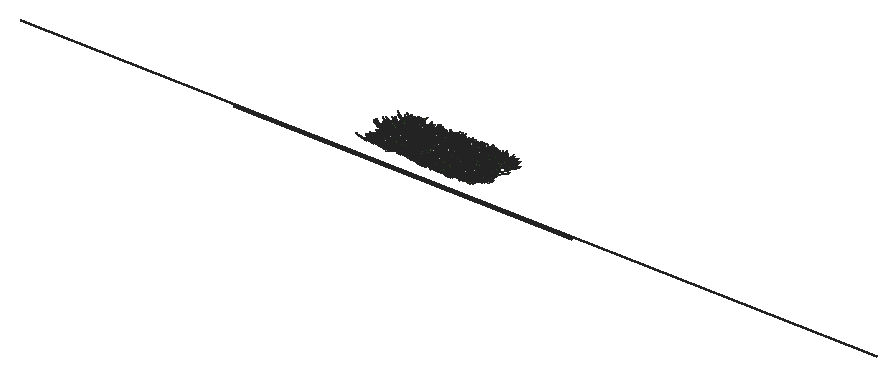
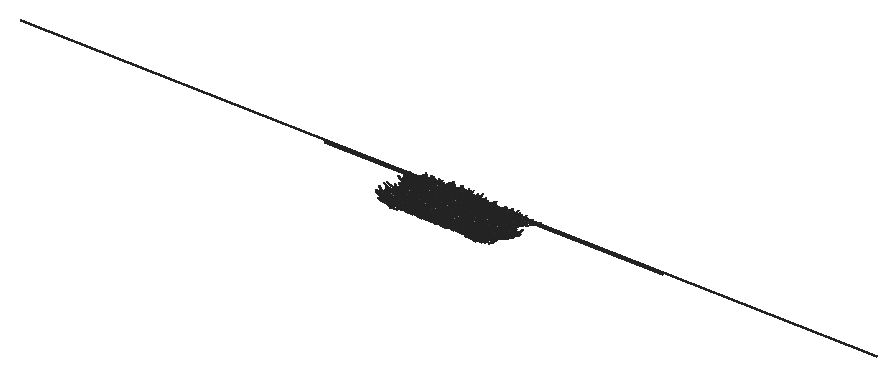
# SketchUp Ruby script. Lengths in inches.
U = 1.inch
M = Sketchup.active_model
def pt(a) = Geom::Point3d.new(a.map { |v| v * U })
def face(e, loops, mat)
  f = e.add_face(loops[0].map { |a| pt(a) })
  loops[1..].each { |l| e.add_face(l.map { |a| pt(a) }).erase! }
  f.material = f.back_material = mat if mat
  f
end
# faces: each face lists its corners as indices into pts; further lists are holes
def faces(e, pts, list, mat = nil) = list.each { |f| face(e, (f[0].is_a?(Array) ? f : [f]).map { |l| l.map { |i| pts[i] } }, mat) }
# xy, xz, yz: faces in a plane at the given z, y or x. An outline is a flat list of corners, or four numbers for a rectangle; further outlines are holes
def ring(l) = l.size == 4 ? [[l[0], l[1]], [l[2], l[1]], [l[2], l[3]], [l[0], l[3]]] : l.each_slice(2).to_a
def flat(e, list, mat, &to3) = list.each { |f| face(e, (f[0].is_a?(Array) ? f : [f]).map { |l| ring(l).map { |u, v| to3.(u, v) } }, mat) }
def xy(e, z, list, mat = nil) = flat(e, list, mat) { |x, y| [x, y, z] }
def xz(e, y, list, mat = nil) = flat(e, list, mat) { |x, z| [x, y, z] }
def yz(e, x, list, mat = nil) = flat(e, list, mat) { |y, z| [x, y, z] }
def lines(e, pts, list) = list.each { |a, b| e.add_line(pt(pts[a]), pt(pts[b])) }
# prism: a flat outline (further loops are holes) pulled along v
def prism(e, loops, v, mat = nil)
  f = face(e, loops, mat); d = Geom::Vector3d.new(v.map { |x| x * U })
  f.pushpull(f.normal.samedirection?(d) ? d.length : -d.length)
end
def box(e, o, s, mat = nil) = prism(e, [[o, [o[0] + s[0], o[1], o[2]], [o[0] + s[0], o[1] + s[1], o[2]], [o[0], o[1] + s[1], o[2]]]], [0, 0, s[2]], mat)
def at(x, y, z, deg = 0) = Geom::Transformation.translation(pt([x, y, z])) * Geom::Transformation.rotation(ORIGIN, Z_AXIS, deg.degrees)
def axes(o, x, y, z) = Geom::Transformation.new([*x, 0, *y, 0, *z, 0, *pt(o).to_a, 1])
def part(name) = M.definitions.add(name)
# library, detail: a bought-in or finely detailed component or shape, given as its bounding box
def library(name, o, s) = part(name).tap { |d| box(d.entities, o, s) }
def detail(e, o, s) = box(e.add_group.entities, o, s)
def put(e, d, t, mat = nil) = e.add_instance(d, t).tap { |i| i.material = mat if mat }
def group(e, t, mat = nil) = e.add_group.tap { |g| g.transformation = t; g.material = mat if mat }.entities
root = M.entities
M.materials.add("Material82").color = [68, 110, 58]
M.materials.add("Material83").color = [48, 90, 38]
M.materials.add("Material84").color = [68, 110, 48]
M.materials.add("Material85").color = [48, 90, 48]
M.materials.add("Material86").color = [58, 110, 58]
M.materials.add("Material87").color = [58, 90, 38]
M.materials.add("Material88").color = [68, 100, 58]
M.materials.add("Material89").color = [48, 100, 38]
c1 = part("grass00")
p = [[-0.6875,0.15,0],[-0.56,0.08,5.52],[-0.04,0.03,2.76],[0.48,-0.02,0],[0.35,-0.02,5.52],[-0.1,-0.14,5.52],
  [-0.12,0.65,8.37],[-0.42,0.65,8.37]]
faces(c1.entities,p,[[0,1,2,3],[3,2,4],[1,5,2],[5,4,2],[1,6,5],[4,5,6],[7,6,1]])
c2 = part("Group16\#1")
put(c2.entities,c1,axes([1.44,-0.61,-0.01],[0.05352,0.12609,0],[-0.10704,0.04543,0.07239],[0.06664,-0.02828,0.11628]),"Material85")
put(c2.entities,c1,axes([0.76,-0.15,-0.01],[0.04676,0.24062,0],[-0.23162,0.04501,0.06642],[0.0652,-0.01267,0.23595]),"Material82")
put(c2.entities,c1,axes([0.79,0.01,-0.01],[-0.00606,0.34651,0],[-0.34381,-0.00602,0.0432],[0.04319,0.00076,0.34386]))
put(c2.entities,c1,axes([1,0.23,-0.01],[-0.07192,0.31144,0],[-0.28722,-0.06632,0.1236],[0.12043,0.02781,0.29478]),"Material84")
put(c2.entities,c1,axes([1.66,0.77,-0.01],[-0.13828,0.29651,0],[-0.21551,-0.1005,0.22471],[0.20365,0.09498,0.23779]),"Material89")
put(c2.entities,c1,axes([0.6875,0.52,-0.01],[-0.18126,0.24051,0],[-0.22746,-0.17142,0.09788],[0.07817,0.05891,0.28481]),"Material84")
put(c2.entities,c1,axes([0.68,0.78,-0.01],[-0.215,0.18688,0],[-0.12385,-0.14248,0.21334],[0.13995,0.16101,0.18878]),"Material82")
put(c2.entities,c1,axes([0.56,1,-0.01],[-0.13756,0.07624,0],[-0.06159,-0.11112,0.0927],[0.04494,0.08108,0.12705]),"Material84")
put(c2.entities,c1,axes([0.2,0.64,-0.01],[-0.23729,0.07254,0],[-0.05711,-0.18681,0.153],[0.04473,0.14632,0.19535]),"Material89")
put(c2.entities,c1,axes([0.0625,0.72,-0.01],[-0.28874,0.02525,0],[-0.02179,-0.24916,0.14647],[0.01276,0.14591,0.25012]),"Material82")
put(c2.entities,c1,axes([-0.08,0.62,-0.01],[-0.34089,-0.04187,0],[0.03255,-0.26504,0.216],[-0.02633,0.21439,0.26703]),"Material89")
put(c2.entities,c1,axes([-0.34,0.98,-0.01],[-0.14314,-0.0493,0],[0.04397,-0.12769,0.06843],[-0.02228,0.0647,0.13505]),"Material89")
put(c2.entities,c1,axes([-0.87,1.45,-0.01],[-0.23488,-0.14114,0],[0.13761,-0.22901,0.06087],[-0.03135,0.05217,0.26717]))
put(c2.entities,c1,axes([-0.72,0.77,-0.01],[-0.14208,-0.13251,0],[0.07209,-0.0773,0.16301],[-0.11118,0.11922,0.1057]),"Material89")
put(c2.entities,c1,axes([-0.62,0.43,-0.01],[-0.14845,-0.21203,0],[0.18654,-0.13061,0.12304],[-0.10079,0.07057,0.22772]),"Material82")
put(c2.entities,c1,axes([-0.68,0.29,-0.01],[-0.13639,-0.32136,0],[0.31723,-0.13464,0.05579],[-0.05136,0.0218,0.34462]),"Material83")
put(c2.entities,c1,axes([-0.64,0.125,-0.01],[-0.0458,-0.23569,0],[0.22124,-0.043,0.08276],[-0.08124,0.01579,0.22538]),"Material86")
put(c2.entities,c1,axes([-1.6,-0.03,-0.01],[0.00576,-0.32897,0],[0.27526,0.00482,0.18018],[-0.18015,-0.00315,0.2753]),"Material84")
put(c2.entities,c1,axes([-1.36,-0.31,-0.01],[0.05718,-0.24765,0],[0.18172,0.04196,0.17267],[-0.16825,-0.03885,0.1865]),"Material89")
put(c2.entities,c1,axes([-1.54,-0.72,-0.01],[0.06537,-0.14017,0],[0.13555,0.06321,0.03939],[-0.0357,-0.01665,0.14956]))
put(c2.entities,c1,axes([-1.19,-0.9,-0.01],[0.09597,-0.12735,0],[0.11214,0.08451,0.07557],[-0.06035,-0.04548,0.14042]),"Material88")
put(c2.entities,c1,axes([-0.47,-0.54,-0.01],[0.11588,-0.10072,0],[0.0618,0.0711,0.12124],[-0.07953,-0.0915,0.0942]))
put(c2.entities,c1,axes([-0.47,-0.84,-0.01],[0.11927,-0.0661,0],[0.06603,0.11913,0.00646],[-0.00313,-0.00565,0.13621]),"Material84")
put(c2.entities,c1,axes([-0.38,-1.24,-0.01],[0.28037,-0.08571,0],[0.0618,0.20215,0.20315],[-0.05939,-0.19428,0.21139]),"Material88")
put(c2.entities,c1,axes([-0.06,-0.66,-0.01],[0.22719,-0.01987,0],[0.01247,0.14255,0.17758],[-0.01547,-0.17691,0.1431]),"Material87")
put(c2.entities,c1,axes([0.11,-0.89,-0.01],[0.14882,0.01828,0],[-0.01058,0.08611,0.12229],[0.01491,-0.12138,0.08676]),"Material85")
put(c2.entities,c1,axes([0.25,-0.72,-0.01],[0.20481,0.07053,0],[-0.06206,0.18022,0.10291],[0.03351,-0.0973,0.1906]),"Material85")
put(c2.entities,c1,axes([0.85,-1.42,-0.01],[0.16481,0.09904,0],[-0.09472,0.15762,0.05616],[0.02893,-0.04814,0.18389]),"Material84")
put(c2.entities,c1,axes([1.01,-1.09,-0.01],[0.21858,0.20385,0],[-0.17495,0.1876,0.15339],[0.10462,-0.11218,0.25652]),"Material89")
put(c2.entities,c1,axes([1.01,-0.71,-0.01],[0.08733,0.12473,0],[-0.06445,0.04512,0.13037],[0.1068,-0.07477,0.07867]),"Material85")
c3 = part("Group15\#1")
put(c3.entities,c2,at(0,0,0))
c4 = part("3darcstudiotree_grass00\#1")
put(c4.entities,c3,at(0,0,0))
xz(root,273.41,[[1674.99,-39.125,1897.28,-38.61],[1534.73,-37.86,2096.97,-37.24]])
put(root,c4,axes([1803.56,281.3125,-34.17],[3.22982,-1.36398,0],[2.52221,0.92889,-0.01281],[0.05669,0.02088,1.56626]))
put(root,c4,axes([1811.6875,281.07,-34.17],[0.45304,1.69594,0],[-3.37186,0.14009,-0.01763],[-0.11097,0.00461,1.60818]))
put(root,c4,axes([1801.04,281.26,-34.17],[-2.98133,1.10226,0],[-2.6348,-1.10837,-0.04557],[-0.21161,-0.08902,1.96028]))
put(root,c4,axes([1793.37,281.49,-34.17],[0.75696,1.65896,0],[-4.64105,0.32936,-0.03105],[-0.12997,0.00922,1.50318]))
put(root,c4,axes([1821.67,281.36,-34.17],[-1.86859,1.14232,0],[-3.14905,-0.80116,-0.00439],[-0.02189,-0.00557,1.66469]))
put(root,c4,axes([1767.47,282.96,-34.17],[3.31562,-0.63662,0],[1.81859,1.47309,-0.02466],[0.05194,0.04207,1.49812]))
put(root,c4,axes([1817.85,282.6,-34.17],[2.60331,1.05125,0],[-2.58261,0.9947,-0.01838],[-0.08057,0.03103,1.65818]))
put(root,c4,axes([1783.02,282.9375,-34.17],[4.09444,0.12503,0],[-0.31641,1.61154,-0.0417],[-0.02006,0.10219,1.91485]))
put(root,c4,axes([1804.3,283.15,-34.17],[3.14565,-0.76847,0],[1.85222,1.17921,-0.00486],[0.01386,0.00882,1.42853]))
put(root,c4,axes([1786.66,282.67,-34.17],[-0.14266,1.36173,0],[-4.10184,-0.06683,-0.00296],[-0.01424,-0.00023,1.47961]))
put(root,c4,axes([1770.84,282.6,-34.17],[-3.65106,0.9561,0],[-2.55118,-1.5152,-0.05111],[-0.12576,-0.07469,1.53759]))
put(root,c4,axes([1798.7,282.95,-34.17],[-3.45178,0.2701,0],[-0.90786,-1.80446,-0.05548],[-0.0508,-0.10098,1.6451]))
put(root,c4,axes([1775.57,283.58,-34.17],[3.35024,-0.43777,0],[1.10858,1.31952,-0.03222],[0.06859,0.08164,1.78787]))
put(root,c4,axes([1762.07,283.2,-34.17],[-4.08016,-0.15242,0],[0.34321,-1.42893,-0.02721],[0.0124,-0.05162,1.31849]))
put(root,c4,axes([1820.89,283.29,-34.17],[-0.10583,1.54224,0],[-3.7996,-0.04055,-0.00627],[-0.03571,-0.00038,1.62459]))
put(root,c4,axes([1792.28,283.65,-34.17],[-2.56709,-0.87628,0],[2.75862,-1.25691,-0.00422],[0.01164,-0.0053,1.33295]))
put(root,c4,axes([1810.66,283.9,-34.17],[2.94971,1.39882,0],[-3.26889,1.07209,-0.02991],[-0.14108,0.04627,1.95467]))
put(root,c4,axes([1787.83,284.71,-34.17],[3.68364,0.44666,0],[-1.28613,1.64968,-0.02064],[-0.02718,0.03487,1.46981]))
put(root,c4,axes([1804.67,285.1,-34.17],[1.53079,-1.5017,0],[4.19952,0.6658,-0.01772],[0.08663,0.01374,1.7874]))
put(root,c4,axes([1765.65,284.68,-34.17],[-0.8053,1.43922,0],[-4.1788,-0.36366,-0.05256],[-0.20936,-0.01822,1.30827]))
put(root,c4,axes([1800.85,285.36,-34.17],[1.13972,-1.41461,0],[4.50389,0.56436,-0.03698],[0.18209,0.02282,1.82987]))
put(root,c4,axes([1782.94,285.26,-34.17],[3.61655,0.77067,0],[-2.16585,1.58076,-0.05913],[-0.11484,0.08382,1.39517]))
put(root,c4,axes([1794.16,285.29,-34.17],[-1.56362,-1.21345,0],[3.6466,-0.73082,-0.00876],[0.03709,-0.00743,1.45672]))
put(root,c4,axes([1823.15,285.4,-34.17],[-3.61232,0.8121,0],[-2.24589,-1.55373,-0.01918],[-0.05035,-0.03483,1.80194]))
put(root,c4,axes([1814.34,286.01,-34.17],[3.57437,0.42668,0],[-1.04232,1.35805,-0.0422],[-0.08519,0.111,1.87907]))
put(root,c4,axes([1776.02,286.11,-34.17],[2.52987,0.96809,0],[-2.35442,0.95693,-0.00683],[-0.03278,0.01332,1.74693]))
put(root,c4,axes([1773,285.88,-34.17],[0.40934,1.39565,0],[-3.638,0.16595,-0.04522],[-0.26335,0.01201,1.60941]))
put(root,c4,axes([1812.32,285.87,-34.17],[-3.36311,0.85521,0],[-1.93534,-1.1837,-0.01497],[-0.0443,-0.0271,1.4615]))
put(root,c4,axes([1817.17,286.72,-34.17],[-0.65586,-1.46962,0],[4.60144,-0.31938,-0.05842],[0.32577,-0.02261,1.98292]))
put(root,c4,axes([1826.3,286.73,-34.17],[-3.01218,-1.1682,0],[2.32929,-0.93411,-0.00764],[0.03903,-0.01565,1.81511]))
put(root,c4,axes([1776.07,286.96,-34.17],[0.10079,1.33733,0],[-4.05045,0.04748,-0.05613],[-0.28184,0.0033,1.5259]))
put(root,c4,axes([1821.84,287.11,-34.17],[-0.80891,1.58211,0],[-4.50454,-0.3582,-0.03197],[-0.1625,-0.01292,1.78572]))
put(root,c4,axes([1811.23,287.18,-34.17],[-2.18902,1.07825,0],[-2.9207,-0.92221,-0.02462],[-0.13408,-0.04234,1.95656]))
put(root,c4,axes([1769.99,287.61,-34.17],[-2.79747,-0.82267,0],[2.4,-1.26929,-0.00029],[0.00098,-0.00052,1.69542]))
put(root,c4,axes([1795.17,287.51,-34.17],[0.20899,1.64265,0],[-4.27343,0.08456,-0.03261],[-0.1888,0.00374,1.85888]))
put(root,c4,axes([1784,287.79,-34.17],[-3.83423,-0.51133,0],[1.38691,-1.61748,-0.06149],[0.1095,-0.1277,1.80385]))
put(root,c4,axes([1806.43,288.25,-34.17],[0.38628,-1.42854,0],[3.50239,0.14729,-0.04937],[0.32013,0.01346,1.72169]))
put(root,c4,axes([1766.97,287.69,-34.17],[-1.21632,1.56365,0],[-3.36368,-0.40694,-0.03727],[-0.21338,-0.02582,1.57911]))
put(root,c4,axes([1789.53,287.77,-34.17],[-2.10873,0.99525,0],[-2.92476,-0.96381,-0.03387],[-0.14037,-0.04626,1.54303]))
put(root,c4,axes([1781.45,289.03,-34.17],[4.32757,-0.42653,0],[1.12297,1.77206,-0.03338],[0.0321,0.05066,1.37691]))
put(root,c4,axes([1801.32,288.3,-34.17],[-3.3677,0.38425,0],[-1.22656,-1.67195,-0.00573],[-0.0077,-0.0105,1.59925]))
put(root,c4,axes([1798.86,289.42,-34.17],[4.24203,-0.02956,0],[0.08072,1.80172,-0.02875],[0.00231,0.05162,1.55972]))
put(root,c4,axes([1779.08,289.23,-34.17],[-2.64283,-1.13535,0],[3.48014,-1.25993,-0.02326],[0.08818,-0.03192,1.82249]))
put(root,c4,axes([1816.71,289.62,-34.17],[1.16933,-1.48396,0],[3.883,0.47588,-0.02169],[0.1048,0.01284,1.54236]))
put(root,c4,axes([1804.05,289.61,-34.17],[3.86384,0.07818,0],[-0.23972,1.84255,-0.05168],[-0.01275,0.09801,1.68853]))
put(root,c4,axes([1789.375,289.94,-34.17],[3.33633,-0.58263,0],[1.85643,1.65335,-0.04981],[0.10311,0.09183,1.75709]))
put(root,c4,axes([1766.5,290.5,-34.17],[2.313,-1.43442,0],[2.99954,0.75225,-0.04064],[0.1888,0.04735,1.46692]))
put(root,c4,axes([1821.45,290.52,-34.17],[0.21445,-1.64927,0],[3.6182,0.07317,-0.01161],[0.06174,0.00125,1.44612]))
put(root,c4,axes([1792.65,290.38,-34.17],[2.09092,1.38555,0],[-3.43654,0.80658,-0.00188],[-0.01015,0.00238,1.87843]))
put(root,c4,axes([1811.67,290.52,-34.17],[-2.42754,-1.16571,0],[2.71881,-0.88058,-0.021],[0.08634,-0.02796,1.40308]))
put(root,c4,axes([1773.4,290.24,-34.17],[-2.97215,1.15542,0],[-3.15373,-1.26173,-0.01243],[-0.04576,-0.01831,1.76595]))
put(root,c4,axes([1812.72,291.39,-34.17],[3.8213,1.10557,0],[-2.37941,1.27911,-0.00415],[-0.01079,0.0058,1.32509]))
put(root,c4,axes([1766.01,291.5,-34.17],[3.43029,0.99275,0],[-1.97308,1.06035,-0.01519],[-0.04853,0.02608,1.34969]))
put(root,c4,axes([1820.98,291.5,-34.17],[-3.1974,-0.52057,0],[1.31873,-1.25975,-0.01181],[0.03016,-0.02882,1.73426]))
put(root,c4,axes([1800.07,291.51,-34.17],[-3.96689,-0.26306,0],[0.64548,-1.51387,-0.0114],[0.01279,-0.03,1.97478]))
put(root,c4,axes([1792.88,292.32,-34.17],[3.4734,-0.75241,0],[2.06047,1.47936,-0.02691],[0.07219,0.05183,1.78778]))
put(root,c4,axes([1778.53,292.4375,-34.17],[1.26532,-1.44178,0],[3.12553,0.42661,-0.00044],[0.00223,0.0003,1.32507]))
put(root,c4,axes([1769.97,292.03,-34.17],[2.61816,1.29298,0],[-2.60516,0.82044,-0.01421],[-0.06264,0.01973,1.40932]))
put(root,c4,axes([1787.01,292.6,-34.17],[2.17735,-1.14497,0],[3.55677,1.05197,-0.03529],[0.11494,0.03399,1.35654]))
put(root,c4,axes([1784.36,291.86,-34.17],[-3.45507,0.18922,0],[-0.60525,-1.7188,-0.02154],[-0.01288,-0.03658,1.4342]))
put(root,c4,axes([1806.86,291.99,-34.17],[0.41177,1.61489,0],[-3.5087,0.13914,-0.04963],[-0.27633,0.01096,1.47912]))
put(root,c4,axes([1816.5,292.23,-34.17],[-3.24054,-0.28468,0],[0.77392,-1.37016,-0.02543],[0.03342,-0.05916,1.61262]))
put(root,c4,axes([1778.15,293.65,-34.17],[3.40614,0.32781,0],[-0.81542,1.31776,-0.01459],[-0.02356,0.03807,1.75568]))
put(root,c4,axes([1823.04,293.92,-34.17],[4.64374,0.18316,0],[-0.43015,1.69615,-0.02551],[-0.01161,0.04577,1.48132]))
put(root,c4,axes([1789.8125,293.4,-34.17],[-3.50392,-0.27669,0],[0.88512,-1.7433,-0.02406],[0.02146,-0.04227,1.53532]))
put(root,c4,axes([1783.75,293.52,-34.17],[1.33968,1.52005,0],[-3.16755,0.43419,-0.01128],[-0.07711,0.01057,1.81963]))
put(root,c4,axes([1814.71,294.16,-34.17],[1.53865,-1.45346,0],[4.25105,0.69992,-0.03949],[0.18935,0.03118,1.7941]))
put(root,c4,axes([1769.93,294,-34.17],[-3.43052,-0.93956,0],[2.00829,-1.14045,-0.00375],[0.01479,-0.0084,1.82358]))
put(root,c4,axes([1798.24,294.53,-34.17],[-0.8562,-1.46222,0],[3.2715,-0.29793,-0.0292],[0.1741,-0.01586,1.53984]))
put(root,c4,axes([1805.19,294.38,-34.17],[-3.12873,-1.31633,0],[2.88309,-1.0658,-0.03051],[0.12402,-0.04585,1.65027]))
put(root,c4,axes([1764.82,294.17,-34.17],[1.08587,1.67228,0],[-4.264,0.43062,-0.00469],[-0.02209,0.00223,1.60422]))
put(root,c4,axes([1762.11,294.57,-34.17],[-2.42435,1.35441,0],[-3.23148,-0.89962,-0.04566],[-0.20763,-0.0578,1.65042]))
put(root,c4,axes([1795.18,294.8,-34.17],[-2.97303,0.61552,0],[-2.04085,-1.53313,-0.02543],[-0.06857,-0.05151,1.9093]))
put(root,c4,axes([1777.9375,295.45,-34.17],[0.04452,-1.40138,0],[3.5701,0.01764,-0.00992],[0.04898,0.00024,1.32167]))
put(root,c4,axes([1811.77,294.86,-34.17],[-4.30499,0.20084,0],[-0.50439,-1.68151,-0.02284],[-0.01208,-0.04026,1.44864]))
put(root,c4,axes([1801.41,295.68,-34.17],[-2.49551,-1.26471,0],[2.8619,-0.87828,-0.01663],[0.09126,-0.02801,1.89037]))
put(root,c4,axes([1782.125,296,-34.17],[3.17214,0.39156,0],[-1.05658,1.33127,-0.01935],[-0.04192,0.05282,1.92273]))
put(root,c4,axes([1760.46,296.01,-34.17],[3.52761,0.55067,0],[-1.26989,1.26523,-0.04887],[-0.1287,0.12823,1.85053]))
put(root,c4,axes([1768.47,296.8,-34.17],[3.22727,-0.96219,0],[2.40393,1.25403,-0.04167],[0.15655,0.08166,1.86151]))
put(root,c4,axes([1814.26,296.79,-34.17],[1.36885,-1.43158,0],[3.98655,0.59286,-0.04892],[0.27754,0.04127,1.93615]))
put(root,c4,axes([1809.48,296.19,-34.17],[-3.9685,0.8355,0],[-2.02289,-1.49439,-0.03463],[-0.09424,-0.06962,1.86049]))
put(root,c4,axes([1773.5,296.36,-34.17],[1.39622,1.62786,0],[-3.6301,0.48424,-0.04556],[-0.23124,0.03085,1.53888]))
put(root,c4,axes([1787.88,296.34,-34.17],[-4.01589,0.275,0],[-0.74615,-1.69466,-0.05401],[-0.03733,-0.08478,1.3206]))
put(root,c4,axes([1822.04,296.38,-34.17],[-3.10318,1.24143,0],[-2.60712,-1.01358,-0.05097],[-0.2393,-0.09303,1.80901]))
put(root,c4,axes([1803.88,296.39,-34.17],[0.17144,1.84869,0],[-4.60552,0.06643,-0.0182],[-0.07619,0.0011,1.44668]))
put(root,c4,axes([1794.84,296.81,-34.17],[2.02269,1.40625,0],[-2.88305,0.64496,-0.03898],[-0.27125,0.06068,1.98748]))
put(root,c4,axes([1765.61,297.63,-34.17],[0.48715,-1.38403,0],[3.63737,0.19912,-0.0013],[0.00869,0.00048,1.85519]))
put(root,c4,axes([1822.52,297.67,-34.17],[4.4529,0.04613,0],[-0.09862,1.48061,-0.04419],[-0.00818,0.12282,1.98467]))
put(root,c4,axes([1811.61,297.87,-34.17],[-1.73285,-1.40976,0],[3.20349,-0.61242,-0.03263],[0.20579,-0.03934,1.87]))
put(root,c4,axes([1789.68,297.76,-34.17],[0.25957,1.50579,0],[-3.94932,0.10588,-0.02807],[-0.1244,0.00334,1.3177]))
put(root,c4,axes([1778.29,298.47,-34.17],[3.60093,0.62069,0],[-1.54425,1.39338,-0.01451],[-0.03218,0.02903,1.59989]))
put(root,c4,axes([1817.85,298.41,-34.17],[-3.57377,-0.68668,0],[1.88387,-1.52489,-0.02869],[0.074,-0.0599,1.89824]))
put(root,c4,axes([1770.88,298.84,-34.17],[4.25337,0.6683,0],[-1.56461,1.54873,-0.01606],[-0.02903,0.02874,1.54782]))
put(root,c4,axes([1792.18,298.39,-34.17],[-2.10864,1.34219,0],[-3.56504,-0.87109,-0.01218],[-0.05259,-0.01285,1.59607]))
put(root,c4,axes([1781.2,298.36,-34.17],[-2.73949,1.39402,0],[-3.69271,-1.12865,-0.03455],[-0.12332,-0.03769,1.58129]))
put(root,c4,axes([1762.34,298.57,-34.17],[-4.29343,-0.7683,0],[1.85419,-1.61153,-0.00153],[0.00342,-0.00297,1.82565]))
put(root,c4,axes([1798.85,299.13,-34.17],[-0.26486,1.49696,0],[-3.89065,-0.10706,-0.02357],[-0.1242,-0.00342,1.54387]))
put(root,c4,axes([1766.81,299.89,-34.17],[2.27709,-1.12887,0],[2.96357,0.92974,-0.01848],[0.07518,0.02359,1.47553]))
put(root,c4,axes([1805.55,299.24,-34.17],[-3.19374,0.7238,0],[-2.32014,-1.59223,-0.04948],[-0.1132,-0.07768,1.60238]))
put(root,c4,axes([1803.55,300.34,-34.17],[4.72899,0.01401,0],[-0.03317,1.74196,-0.012],[-0.00046,0.02441,1.70791]))
put(root,c4,axes([1781.52,300.48,-34.17],[-2.29669,-1.11112,0],[2.95834,-0.95105,-0.00371],[0.01505,-0.00484,1.4993]))
put(root,c4,axes([1794.4,300.5,-34.17],[-3.17921,-1.35137,0],[3.1644,-1.15784,-0.01209],[0.04457,-0.01631,1.62724]))
put(root,c4,axes([1820.83,300.76,-34.17],[-0.51556,-1.46046,0],[3.95081,-0.21691,-0.04493],[0.28513,-0.01565,1.91565]))
put(root,c4,axes([1816.55,300.875,-34.17],[-1.16799,-1.2811,0],[3.57696,-0.50721,-0.0171],[0.1013,-0.01436,1.79343]))
put(root,c4,axes([1812.14,300.54,-34.17],[0.87217,1.79185,0],[-4.36686,0.33058,-0.02457],[-0.1156,0.00875,1.59681]))
put(root,c4,axes([1762.38,301.35,-34.17],[0.26653,-1.73376,0],[4.03869,0.09656,-0.02606],[0.1443,0.00345,1.68211]))
put(root,c4,axes([1798.5,301.02,-34.17],[-4.0045,-0.70324,0],[1.53901,-1.36302,-0.04343],[0.08424,-0.0746,1.35201]))
put(root,c4,axes([1779.39,301.04,-34.17],[-0.93158,1.57452,0],[-3.64716,-0.33561,-0.02125],[-0.09909,-0.00912,1.34411]))
put(root,c4,axes([1787.33,301.15,-34.17],[-1.92395,1.11114,0],[-2.73961,-0.73778,-0.01899],[-0.11099,-0.02989,1.75992]))
put(root,c4,axes([1774,302.05,-34.17],[4.28281,-0.63976,0],[1.42181,1.48036,-0.01068],[0.01649,0.01717,1.31138]))
put(root,c4,axes([1770.08,301.36,-34.17],[-3.74102,0.70585,0],[-1.92999,-1.5909,-0.05113],[-0.08819,-0.0727,1.33965]))
put(root,c4,axes([1816.35,302.07,-34.17],[4.39904,-0.03006,0],[0.06093,1.38656,-0.04649],[0.00481,0.10943,1.57333]))
put(root,c4,axes([1797.97,302.36,-34.17],[2.12424,-1.58648,0],[2.98317,0.62124,-0.03491],[0.20173,0.04201,1.65255]))
put(root,c4,axes([1790.23,302.7,-34.17],[2.84805,-1.35819,0],[2.78081,0.90692,-0.04304],[0.21584,0.07039,1.76026]))
put(root,c4,axes([1793.73,302.4,-34.17],[-1.97289,1.32597,0],[-3.97358,-0.91953,-0.01374],[-0.05147,-0.01191,1.50009]))
put(root,c4,axes([1779.05,302.52,-34.17],[-4.13794,-0.2249,0],[0.58111,-1.66288,-0.00876],[0.00496,-0.01418,1.32289]))
put(root,c4,axes([1803.68,302.74,-34.17],[1.47307,1.52241,0],[-3.55442,0.5349,-0.03212],[-0.18221,0.02742,1.73128]))
put(root,c4,axes([1765.14,302.92,-34.17],[-4.03021,-0.53258,0],[1.1352,-1.33605,-0.02118],[0.04192,-0.04934,1.66873]))
put(root,c4,axes([1819.98,303.0625,-34.17],[-4.17671,-0.8199,0],[2.05439,-1.62767,-0.0574],[0.10467,-0.08292,1.41402]))
put(root,c4,axes([1809.0625,303.1,-34.17],[-1.70053,1.52985,0],[-3.13018,-0.54115,-0.01229],[-0.08699,-0.01504,1.9803]))
put(root,c4,axes([1784.3125,303.53,-34.17],[-0.83712,1.35251,0],[-3.5635,-0.34303,-0.03757],[-0.17469,-0.01682,1.3158]))
put(root,c4,axes([1823.19,304.51,-34.17],[1.76506,-1.25364,0],[3.37171,0.73833,-0.03203],[0.17156,0.03757,1.771]))
put(root,c4,axes([1766.34,304.68,-34.17],[4.01997,0.45296,0],[-1.05214,1.45226,-0.01128],[-0.01738,0.02399,1.61003]))
put(root,c4,axes([1817.7,304.58,-34.17],[-3.73914,-0.79189,0],[1.71097,-1.25649,-0.0264],[0.09118,-0.06696,1.979]))
put(root,c4,axes([1794.46,304.67,-34.17],[-2.5712,-1.27561,0],[3.33499,-1.0455,-0.01168],[0.0385,-0.01207,1.34439]))
put(root,c4,axes([1773.42,305.08,-34.17],[-1.28823,-1.73919,0],[3.44626,-0.39701,-0.03009],[0.18497,-0.02131,1.72353]))
put(root,c4,axes([1801.19,305.2,-34.17],[4.6709,-0.11713,0],[0.23839,1.47848,-0.03177],[0.01367,0.08477,1.90853]))
put(root,c4,axes([1806.67,304.68,-34.17],[-1.61807,1.52118,0],[-3.6405,-0.60227,-0.04701],[-0.26943,-0.04457,1.83905]))
put(root,c4,axes([1812.51,305.29,-34.17],[0.02605,-1.38879,0],[4.64619,0.01356,-0.04606],[0.23946,0.0007,1.81052]))
put(root,c4,axes([1787.94,305.15,-34.17],[-4.087,-0.33484,0],[0.93219,-1.7696,-0.02537],[0.02744,-0.05209,1.82613]))
put(root,c4,axes([1785.07,305.8,-34.17],[3.08356,-0.59749,0],[1.85245,1.48689,-0.05746],[0.15906,0.12767,1.97658]))
put(root,c4,axes([1775.89,305.67,-34.17],[-1.97401,-1.44609,0],[3.51216,-0.74566,-0.02018],[0.11603,-0.02463,1.95264]))
put(root,c4,axes([1821.24,306.49,-34.17],[3.31436,0.96989,0],[-2.30719,1.22623,-0.02502],[-0.09786,0.05201,1.90511]))
put(root,c4,axes([1825.61,306.87,-34.17],[1.677,-1.55355,0],[4.28787,0.71988,-0.03539],[0.14144,0.02375,1.51703]))
put(root,c4,axes([1779.27,306.57,-34.17],[1.53583,1.49996,0],[-3.93703,0.62697,-0.05886],[-0.22971,0.03658,1.33951]))
put(root,c4,axes([1800.46,306.44,-34.17],[-3.7951,0.9119,0],[-2.12877,-1.37789,-0.05764],[-0.17628,-0.1141,1.8024]))
put(root,c4,axes([1786.92,306.49,-34.17],[-0.37072,1.84099,0],[-4.27519,-0.13389,-0.01448],[-0.06545,-0.00205,1.45727]))
put(root,c4,axes([1810.9375,307.01,-34.17],[3.34775,0.73741,0],[-1.81639,1.28251,-0.02091],[-0.0568,0.0401,1.55496]))
put(root,c4,axes([1766.66,307.36,-34.17],[4.2861,-0.44175,0],[0.90749,1.36943,-0.02428],[0.0455,0.06867,1.99391]))
put(root,c4,axes([1805.02,307.12,-34.17],[-1.61628,-1.19973,0],[3.67441,-0.7699,-0.00698],[0.03732,-0.00782,1.8873]))
put(root,c4,axes([1781.26,306.72,-34.17],[-2.8718,1.45727,0],[-2.81901,-0.86401,-0.03149],[-0.12433,-0.03811,1.33797]))
put(root,c4,axes([1771.43,307.03,-34.17],[-0.09975,1.34747,0],[-4.08432,-0.04703,-0.00454],[-0.02466,-0.00028,1.66362]))
put(root,c4,axes([1795.02,307.62,-34.17],[1.08869,1.44245,0],[-3.40274,0.39943,-0.00785],[-0.05372,0.00631,1.89978]))
put(root,c4,axes([1815.37,307.93,-34.17],[-2.53143,-1.15701,0],[3.22557,-1.09761,-0.03179],[0.10043,-0.03417,1.33245]))
put(root,c4,axes([1776.79,308.66,-34.17],[3.01451,-0.88182,0],[2.30556,1.22582,-0.02804],[0.08966,0.04767,1.55696]))
put(root,c4,axes([1814.76,308.59,-34.17],[4.54472,-0.07638,0],[0.17813,1.64846,-0.04096],[0.00957,0.08859,1.72127]))
put(root,c4,axes([1789.21,308.76,-34.17],[-0.69027,-1.34957,0],[4.18043,-0.33255,-0.04603],[0.23408,-0.01862,1.65834]))
put(root,c4,axes([1797.92,308.78,-34.17],[3.97101,0.68213,0],[-1.55734,1.41002,-0.04191],[-0.07595,0.06876,1.32656]))
put(root,c4,axes([1784.37,308.65,-34.17],[-3.97452,0.57658,0],[-1.26948,-1.361,-0.04924],[-0.12234,-0.13116,1.98345]))
put(root,c4,axes([1805.33,309.19,-34.17],[3.23921,0.6316,0],[-1.61427,1.28761,-0.03066],[-0.08714,0.06951,1.75054]))
put(root,c4,axes([1794.51,309.04,-34.17],[-3.47552,-0.34069,0],[1.08655,-1.72393,-0.01735],[0.02109,-0.03347,1.70162]))
put(root,c4,axes([1770.8,309.39,-34.17],[-2.1448,1.18286,0],[-3.37437,-0.95161,-0.05929],[-0.21963,-0.06194,1.41608]))
put(root,c4,axes([1765.9,310.01,-34.17],[2.25028,1.20461,0],[-3.26486,0.94856,-0.0323],[-0.12798,0.03718,1.496]))
put(root,c4,axes([1819.79,309.84,-34.17],[-2.56609,1.18757,0],[-3.37526,-1.13431,-0.01912],[-0.05922,-0.0199,1.35238]))
